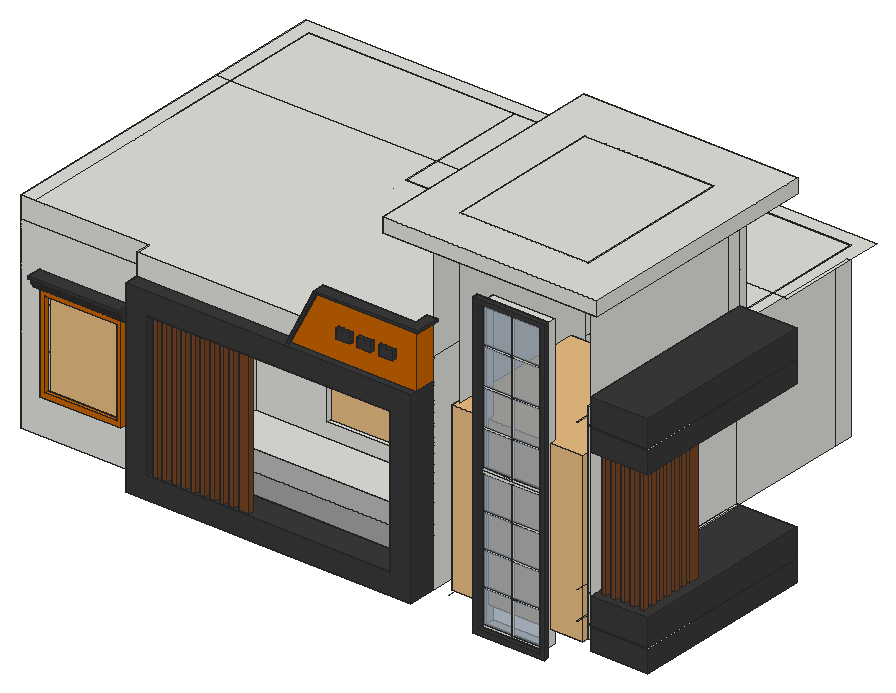
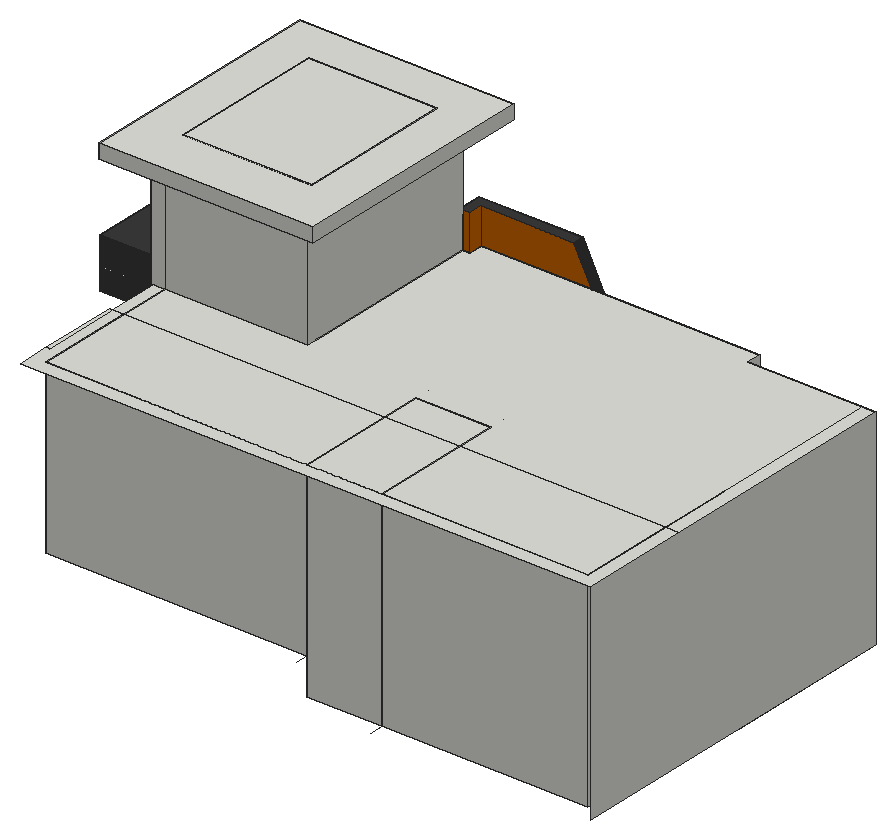
# SketchUp Ruby script. Lengths in inches.
U = 1.inch
M = Sketchup.active_model
def pt(a) = Geom::Point3d.new(a.map { |v| v * U })
def face(e, loops, mat)
  f = e.add_face(loops[0].map { |a| pt(a) })
  loops[1..].each { |l| e.add_face(l.map { |a| pt(a) }).erase! }
  f.material = f.back_material = mat if mat
  f
end
# faces: each face lists its corners as indices into pts; further lists are holes
def faces(e, pts, list, mat = nil) = list.each { |f| face(e, (f[0].is_a?(Array) ? f : [f]).map { |l| l.map { |i| pts[i] } }, mat) }
# xy, xz, yz: faces in a plane at the given z, y or x. An outline is a flat list of corners, or four numbers for a rectangle; further outlines are holes
def ring(l) = l.size == 4 ? [[l[0], l[1]], [l[2], l[1]], [l[2], l[3]], [l[0], l[3]]] : l.each_slice(2).to_a
def flat(e, list, mat, &to3) = list.each { |f| face(e, (f[0].is_a?(Array) ? f : [f]).map { |l| ring(l).map { |u, v| to3.(u, v) } }, mat) }
def xy(e, z, list, mat = nil) = flat(e, list, mat) { |x, y| [x, y, z] }
def xz(e, y, list, mat = nil) = flat(e, list, mat) { |x, z| [x, y, z] }
def yz(e, x, list, mat = nil) = flat(e, list, mat) { |y, z| [x, y, z] }
def lines(e, pts, list) = list.each { |a, b| e.add_line(pt(pts[a]), pt(pts[b])) }
# prism: a flat outline (further loops are holes) pulled along v
def prism(e, loops, v, mat = nil)
  f = face(e, loops, mat); d = Geom::Vector3d.new(v.map { |x| x * U })
  f.pushpull(f.normal.samedirection?(d) ? d.length : -d.length)
end
def box(e, o, s, mat = nil) = prism(e, [[o, [o[0] + s[0], o[1], o[2]], [o[0] + s[0], o[1] + s[1], o[2]], [o[0], o[1] + s[1], o[2]]]], [0, 0, s[2]], mat)
def at(x, y, z, deg = 0) = Geom::Transformation.translation(pt([x, y, z])) * Geom::Transformation.rotation(ORIGIN, Z_AXIS, deg.degrees)
def axes(o, x, y, z) = Geom::Transformation.new([*x, 0, *y, 0, *z, 0, *pt(o).to_a, 1])
def part(name) = M.definitions.add(name)
# library, detail: a bought-in or finely detailed component or shape, given as its bounding box
def library(name, o, s) = part(name).tap { |d| box(d.entities, o, s) }
def detail(e, o, s) = box(e.add_group.entities, o, s)
def put(e, d, t, mat = nil) = e.add_instance(d, t).tap { |i| i.material = mat if mat }
def group(e, t, mat = nil) = e.add_group.tap { |g| g.transformation = t; g.material = mat if mat }.entities
root = M.entities
M.materials.add("[Color C06]").color = [204, 102, 0]
M.materials.add("[Color M07]").color = [58, 58, 58]
M.materials.add("[Marble Carrara Floor Tile]").color = [204, 208, 219]
M.materials.add("[Modern Siding]").color = [191, 132, 100]
M.materials.add("[Polished Concrete New]").color = [200, 200, 203]
M.materials.add("[Stone Vein Gray]").color = [166, 165, 165]
M.materials.add("[Translucent Glass Sky Reflection]").color = [163, 177, 193]
M.materials["[Translucent Glass Sky Reflection]"].alpha = 0.52
M.materials.add("[Wood Floor]").color = [170, 81, 43]
M.materials.add("[Wood Veneer 01]").color = [120, 70, 37]
c1 = part("GLASS WINDOW")
g1 = group(c1.entities,at(60,0,0))
g2 = group(g1,at(-2,0.5,1.97),"[Translucent Glass Sky Reflection]")
box(g2,[-56,0,0],[56,0.75,114.1])
g3 = group(g1,at(0,0,0))
xy(g3,0,[[-60,0,0,2]])
xy(g3,1.97,[[-58,0,-58,2,-2,2,-2,0,-29.5,0,-29.5,1.25,-30.5,1.25,-30.5,0]])
xy(g3,29.75,[[-58,0,-30.5,1.25],[-29.5,0,-2,1.25]])
xy(g3,30.74,[[-58,0,-30.5,1.25],[-29.5,0,-2,1.25]])
xy(g3,58.52,[[-58,0,-30.5,1.25],[-29.5,0,-2,1.25]])
xy(g3,59.51,[[-58,0,-30.5,1.25],[-29.5,0,-2,1.25]])
xy(g3,87.29,[[-58,0,-30.5,1.25],[-29.5,0,-2,1.25]])
xy(g3,88.28,[[-58,0,-30.5,1.25],[-29.5,0,-2,1.25]])
xy(g3,116.0625,[[-58,0,-30.5,0,-30.5,1.25,-29.5,1.25,-29.5,0,-2,0,-2,2,-58,2]])
xy(g3,118.03,[[-60,0,0,2]])
xz(g3,0,[[[-60,0,0,118.03],[-58,59.51,-30.5,87.29],[-58,1.97,-30.5,29.75],[-58,88.28,-30.5,116.0625],[-58,30.74,-30.5,58.52],[-29.5,88.28,-2,116.0625],[-29.5,59.51,-2,87.29],[-29.5,1.97,-2,29.75],[-29.5,30.74,-2,58.52]]])
xz(g3,1.25,[[-30.5,1.97,-29.5,1.97,-29.5,29.75,-2,29.75,-2,30.74,-29.5,30.74,-29.5,58.52,-2,58.52,-2,59.51,-29.5,59.51,-29.5,87.29,-2,87.29,-2,88.28,-29.5,88.28,-29.5,116.0625,-30.5,116.0625,-30.5,88.28,-58,88.28,-58,87.29,-30.5,87.29,-30.5,59.51,-58,59.51,-58,58.52,-30.5,58.52,-30.5,30.74,-58,30.74,-58,29.75,-30.5,29.75]])
xz(g3,2,[[[-60,0,0,118.03],[-58,1.97,-2,116.0625]]])
yz(g3,-60,[[0,0,2,118.03]])
yz(g3,-58,[[0,1.97,0,29.75,1.25,29.75,1.25,30.74,0,30.74,0,58.52,1.25,58.52,1.25,59.51,0,59.51,0,87.29,1.25,87.29,1.25,88.28,0,88.28,0,116.0625,2,116.0625,2,1.97]])
yz(g3,-30.5,[[0,1.97,1.25,29.75],[0,30.74,1.25,58.52],[0,59.51,1.25,87.29],[0,88.28,1.25,116.0625]])
yz(g3,-29.5,[[0,1.97,1.25,29.75],[0,30.74,1.25,58.52],[0,59.51,1.25,87.29],[0,88.28,1.25,116.0625]])
yz(g3,-2,[[0,1.97,2,1.97,2,116.0625,0,116.0625,0,88.28,1.25,88.28,1.25,87.29,0,87.29,0,59.51,1.25,59.51,1.25,58.52,0,58.52,0,30.74,1.25,30.74,1.25,29.75,0,29.75]])
yz(g3,0,[[0,0,2,118.03]])
p = [[-29.5,0,116.0625],[-30.5,0,116.0625]]
lines(g3,p,[[0,1]])
c2 = library("DOG LEGGED STAIRCASE",[0,0,0],[168.93,78,123.9375])
c3 = library("Janela de Correr",[0,0,0],[62.99,2.6,47.24])
xy(root,121.92,[[359.58,113.36,409.62,113.6875]],"[Marble Carrara Floor Tile]")
xy(root,123.09,[[359.58,113.36,409.62,113.6875],[359.58,113.6875,409.62,121.61]],"[Marble Carrara Floor Tile]")
xy(root,126,[[384,20,444,24]],"[Color M07]")
xy(root,128.9,[[359.58,121.28,409.62,121.61]],"[Marble Carrara Floor Tile]")
xy(root,130,[[388,24,440,36]])
xy(root,130,[[388,20,440,24]],"[Color M07]")
xy(root,130.06,[[359.58,121.28,409.62,121.61],[359.58,121.61,409.62,129.53]],"[Marble Carrara Floor Tile]")
xy(root,132,[[24,120,48,184.5625]])
xy(root,135.87,[[359.58,129.2,409.62,129.53]],"[Marble Carrara Floor Tile]")
xy(root,137.03,[[359.58,129.2,409.62,129.53],[359.58,129.53,409.62,137.45]],"[Marble Carrara Floor Tile]")
xy(root,139.43,[[359.58,145.98,468,168]],"[Polished Concrete New]")
xy(root,142.84,[[359.58,137.12,409.62,137.45]],"[Marble Carrara Floor Tile]")
xy(root,144,[[0,24,12,168],[[12,24,12,120,204,120,204,36,192,36,192,24],[162,54,180,66]],[192,24,204,36],[204,24,348,156],[480,24,528,180],
  [468,36,477.125,180],[477.125,36,480,180],[12,120,204,153.875],[359.58,137.12,360,137.45],[359.58,137.45,360,168],
  [12,153.875,204,156],[12,156,348,168],[185.31,168,248.2,180],[348,168,468,180],[12,180,185.31,312],
  [185.31,180,248.2,184.3125],[185.31,184.3125,248.2,197.875],[185.31,197.875,248.2,312]])
xy(root,144,[[108,0,192,24],[192,0,204,24],[204,0,348,24]],"[Color M07]")
xy(root,144,[[360,137.12,409.62,137.45],[360,137.45,409.62,137.45,409.62,145.98,468,145.98,468,168,360,168]],"[Marble Carrara Floor Tile]")
xy(root,162,[[129,2,133,6],[145,2,149,6],[161,2,165,6],[185,2,189,6],[201,2,210,6],
  [126,24,330,48],[480,24,528,180],[126,48,330,114],[126,114,258,204],[258,114,330,114,330,144,328,144,328,148,330,148,330,188,328,188,328,192,330,192,330,204,324,204,324,199,320,199,320,204,273.87,204,273.87,199,270,199,270,204,258,204],
  [328,144,330,148],[328,188,330,192]])
xy(root,162,[[[126,0,330,24],[201,2,210,6],[193,2,197,6],[185,2,189,6],[177,2,181,6],[169,2,173,6],[161,2,165,6],[153,2,157,6],[145,2,149,6],[137,2,141,6],[129,2,133,6]]],"[Color M07]")
xy(root,163,[[480,24,528,180],[477.125,170.25,480,180]])
xy(root,174,[[186,114,246,204]])
xy(root,175.2,[[477.125,170.25,480,170.4375],[477.125,170.4375,480,180]])
xy(root,176,[[20,20,88,24]],"[Color C06]")
xy(root,180,[[24,24,84,143.1875]])
xy(root,180,[[24,20,84,24]],"[Color C06]")
xy(root,180,[[126,24,330,48]],"[Stone Vein Gray]")
xy(root,186,[[484,30,488,34],[500,30,504,34],[516,30,520,34],[516,46,520,50],[516,62,520,66],
  [516,78,520,86],[468,96,477.125,145.98],[477.125,96,480,170.4375],[468,145.98,477.125,168],[468,168,477.125,180],
  [477.125,170.4375,480,180]])
xy(root,186,[[[480,24,528,180],[516,78,520,86],[516,38,520,42],[492,30,496,34],[508,30,512,34],[516,46,520,50],[516,54,520,58],[516,62,520,66],[516,70,520,74],[484,30,488,34],[500,30,504,34],[516,30,520,34]]],"[Color M07]")
xy(root,237.2,[[328,148,330,188]])
xy(root,237.2,[[273.87,199,320,204]],"[Color M07]")
xy(root,241.2,[[186,114,246,204]])
xy(root,241.2,[[328,144,330,192],[270,199,324,204]],"[Color M07]")
xy(root,253.2,[[24,24,84,143.1875]])
xy(root,253.2,[[24,20,84,24]],"[Color C06]")
xy(root,257.2,[[20,20,88,24]],"[Color C06]")
xy(root,257.2,[[16,20,20,24],[88,20,92,24]],"[Color M07]")
xy(root,267.2,[[16,12,92,14]],"[Color M07]")
xy(root,269.2,[[16,12,92,24]],"[Color M07]")
xy(root,281.2,[[264,36,324,192]],"[Modern Siding]")
xy(root,283.2,[[[126,24,126,114,258,114,258,204,330,204,330,24],[264,36,324,192]],[264,36,324,192],[126,114,258,204]])
xy(root,283.2,[[126,0,330,24]],"[Color M07]")
xy(root,294,[[129,2,133,6],[137,2,141,6],[145,2,149,6],[153,2,157,6],[161,2,165,6],
  [169,2,173,6],[177,2,181,6],[185,2,189,6],[193,2,197,6],[201,2,210,6],
  [[480,24,528,180],[516,78,520,86],[516,38,520,42],[516,70,520,74],[516,62,520,66],[516,54,520,58],[516,46,520,50],[508,30,512,34],[492,30,496,34],[484,30,488,34],[516,30,520,34],[500,30,504,34]],[477.125,96,480,168],[477.125,168,480,180]])
xy(root,301.2,[[240,3,240,12,342,12,342,24,348,24,348,6,242.24,6,242.24,3],[108,12,342,24]])
xy(root,301.2,[[108,0,348,0,348,6,242.24,6,242.24,3,240,3,240,12,108,12]],"[Color M07]")
xy(root,312,[[480,24,528,180],[477.125,168,480,180]])
xy(root,313,[[480,24,528,180],[477.125,168,480,180]])
xy(root,319.2,[[108,12,342,12,342,24,348,24,348,187.0625,468,187.0625,468,230.125,248.2,230.125,248.2,197.875,185.31,197.875,185.31,230.125,12,230.125,12,24,108,24],[0,24,12,230.125],[468,36,477.125,187.0625],[477.125,168,480,180],[477.125,180,480,187.0625],
  [468,187.0625,477.125,230.125],[185.31,197.875,248.2,230.125],[0,230.125,12,230.125,12,312,468,312,468,230.125,477.125,230.125,477.125,296.25,480,296.25,480,324,0,324],[12,230.125,185.31,312],[185.31,230.125,248.2,312],
  [248.2,230.125,468,312],[477.125,230.125,480,296.25]])
xy(root,319.2,[[282,3,294,6],[300,3,312,6],[318,3,330,6]],"[Color M07]")
xy(root,327.2,[[282,3,294,6],[300,3,312,6],[318,3,330,6]],"[Color M07]")
xy(root,336,[[480,24,528,180]],"[Color M07]")
xy(root,347.2,[[265.24,3,351,6],[348,6,351,24]],"[Color M07]")
xy(root,349.2,[[264,3,351,3,351,24,342,24,342,12,264,12]],"[Color M07]")
xy(root,375.2,[[388,20,440,24],[388,24,440,36]])
xy(root,379.2,[[384,20,444,24]],"[Color M07]")
xy(root,414.2,[[[328,4,500,207.0625],[342,18,486,193.0625]]],"[Modern Siding]")
xy(root,415.2,[[[324,0,504,211.0625],[328,4,500,207.0625]],[[342,18,486,193.0625],[348,24,480,187.0625]],[[348,24,480,187.0625],[360,36,468,168]],[360,36,468,168]])
xy(root,427.2,[[[324,0,504,211.0625],[360,36,468,168]],[360,36,468,168]])
xz(root,0,[[324,415.2,504,427.2]])
xz(root,0,[[[108,144,348,301.2],[126,162,330,283.2]]],"[Color M07]")
xz(root,2,[[129,162,133,294],[137,162,141,294],[145,162,149,294],[153,162,157,294],[161,162,165,294],
  [169,162,173,294],[177,162,181,294],[185,162,189,294],[193,162,197,294],[201,162,210,294]],"[Wood Veneer 01]")
xz(root,3,[[240,301.2,242.24,301.2,265.24,347.2,351,347.2,351,349.2,264,349.2],[282,319.2,294,327.2],[300,319.2,312,327.2],[318,319.2,330,327.2]],"[Color M07]")
xz(root,4,[[328,414.2,500,415.2]],"[Modern Siding]")
xz(root,6,[[282,319.2,294,327.2],[318,319.2,330,327.2]])
xz(root,6,[[[242.24,301.2,348,301.2,348,347.2,265.24,347.2],[282,319.2,294,327.2],[300,319.2,312,327.2],[318,319.2,330,327.2]]],"[Color C06]")
xz(root,6,[[129,162,133,294],[137,162,141,294],[145,162,149,294],[153,162,157,294],[161,162,165,294],
  [169,162,173,294],[177,162,181,294],[185,162,189,294],[193,162,197,294],[201,162,210,294]],"[Wood Veneer 01]")
xz(root,12,[[108,301.2,240,301.2,249,319.2,108,319.2],[240,301.2,342,301.2,342,319.2,249,319.2]])
xz(root,12,[[249,319.2,264,349.2,342,349.2,342,319.2]],"[Color C06]")
xz(root,12,[[16,267.2,92,269.2]],"[Color M07]")
xz(root,18,[[342,414.2,486,415.2]],"[Modern Siding]")
xz(root,20,[[[20,176,88,257.2],[24,180,84,253.2]]],"[Color C06]")
xz(root,20,[[[384,126,444,379.2],[388,130,440,375.2]]],"[Color M07]")
xz(root,24,[[[384,126,444,379.2],[388,130,440,375.2]],[[0,144,108,301.2],[20,176,20,257.2,16,257.2,16,269.2,92,269.2,92,257.2,88,257.2,88,176]],[[108,144,348,301.2],[126,162,330,283.2]],[[20,176,88,257.2],[24,180,84,253.2]],[16,257.2,92,269.2],
  [0,301.2,108,319.2],[342,301.2,348,319.2],[348,347.2,351,349.2]])
xz(root,24,[[342,319.2,348,349.2]],"[Color C06]")
xz(root,24,[[480,144,528,162],[480,163,528,186],[480,294,528,312],[480,313,528,336]],"[Color M07]")
xz(root,24,[[126,162,330,180]],"[Stone Vein Gray]")
xz(root,30,[[484,186,488,294],[492,186,496,294],[500,186,504,294],[508,186,512,294],[516,186,520,294]],"[Wood Veneer 01]")
xz(root,34,[[484,186,488,294],[492,186,496,294],[500,186,504,294],[508,186,512,294],[516,186,520,294]],"[Wood Veneer 01]")
xz(root,36,[[468,144,477.125,319.2],[360,415.2,468,427.2]])
xz(root,36,[[264,281.2,324,283.2]],"[Modern Siding]")
xz(root,38,[[516,186,520,294]],"[Wood Veneer 01]")
xz(root,42,[[516,186,520,294]],"[Wood Veneer 01]")
xz(root,46,[[516,186,520,294]],"[Wood Veneer 01]")
xz(root,48,[[126,162,330,180]])
xz(root,50,[[516,186,520,294]],"[Wood Veneer 01]")
xz(root,54,[[516,186,520,294]],"[Wood Veneer 01]")
xz(root,58,[[516,186,520,294]],"[Wood Veneer 01]")
xz(root,62,[[516,186,520,294]],"[Wood Veneer 01]")
xz(root,66,[[516,186,520,294]],"[Wood Veneer 01]")
xz(root,70,[[516,186,520,294]],"[Wood Veneer 01]")
xz(root,74,[[516,186,520,294]],"[Wood Veneer 01]")
xz(root,78,[[516,186,520,294]],"[Wood Veneer 01]")
xz(root,86,[[516,186,520,294]],"[Wood Veneer 01]")
xz(root,96,[[477.125,186,480,294]])
xz(root,113.6875,[[359.58,121.92,409.62,123.09]],"[Marble Carrara Floor Tile]")
xz(root,114,[[[126,162,258,283.2],[186,174,246,241.2]]])
xz(root,120,[[60,143,108,144],[108,143,192.6875,144]],"[Color M07]")
xz(root,121.61,[[359.58,123.09,409.62,128.9],[359.58,128.9,409.62,130.06]],"[Marble Carrara Floor Tile]")
xz(root,129.53,[[359.58,130.06,409.62,135.87],[359.58,135.87,409.62,137.03]],"[Marble Carrara Floor Tile]")
xz(root,137.45,[[359.58,137.03,409.62,142.84],[359.58,142.84,409.62,144]],"[Marble Carrara Floor Tile]")
xz(root,143.1875,[[24,180,84,253.2]])
xz(root,144,[[328,162,330,241.2]],"[Color M07]")
xz(root,145.98,[[409.62,139.43,468,144]],"[Polished Concrete New]")
xz(root,148,[[328,162,330,237.2]])
xz(root,168,[[477.125,294,480,312],[477.125,312,480,313],[360,415.2,468,427.2]])
xz(root,170.25,[[477.125,163,480,175.2]])
xz(root,170.4375,[[477.125,175.2,480,186]])
xz(root,180,[[468,144,477.125,162],[477.125,144,480,163],[468,163,477.125,175.2],[477.125,163,480,175.2],[468,175.2,477.125,186],
  [477.125,175.2,480,186],[468,186,477.125,186.125],[468,186.125,477.125,294],[477.125,294,480,312],[477.125,313,480,319.2]])
xz(root,180,[[480,144,528,162],[480,163,528,175.2],[480,175.2,528,186],[480,294,528,312],[480,313,528,319.2],
  [480,319.2,528,336]],"[Color M07]")
xz(root,187.0625,[[348,319.2,468,415.2],[468,319.2,480,415.2]])
xz(root,188,[[328,162,330,237.2]],"[Color M07]")
xz(root,192,[[264,281.2,324,283.2]])
xz(root,192,[[328,162,330,241.2]],"[Color M07]")
xz(root,193.0625,[[342,414.2,486,415.2]],"[Modern Siding]")
xz(root,197.875,[[185.31,144,248.2,319.2]])
xz(root,199,[[270,162,273.87,162,273.87,237.2,320,237.2,320,162,324,162,324,241.2,270,241.2]],"[Color M07]")
xz(root,204,[[[126,162,258,283.2],[186,174,246,241.2]],[258,162,270,162,270,241.2,324,241.2,324,162,330,162,330,283.2,258,283.2]])
xz(root,204,[[273.87,162,320,237.2]],"[Wood Floor]")
xz(root,207.0625,[[328,414.2,500,415.2]],"[Modern Siding]")
xz(root,211.0625,[[324,415.2,504,427.2]])
xz(root,312,[[12,144,185.31,319.2],[185.31,144,248.2,319.2],[248.2,175.2,468,319.2]])
yz(root,0,[[24,144,324,319.2]])
yz(root,12,[[168,144,180,319.2],[180,144,312,319.2]])
yz(root,16,[[20,257.2,19.23,257.67,18.5,258.21,17.83,258.8125,17.21,259.48,16.67,260.2,16.1875,260.97,15.79,261.78,15.46,262.63,15.22,263.5,15.0625,264.39,14.99,265.29,15,266.2,14,267.2,12,267.2,12,269.2,24,269.2,24,257.2]],"[Color M07]")
yz(root,20,[[20,176,24,257.2]],"[Color C06]")
yz(root,24,[[24,180,143.1875,253.2]])
yz(root,24,[[20,180,24,253.2]],"[Color C06]")
yz(root,84,[[24,180,143.1875,253.2]])
yz(root,84,[[20,180,24,253.2]],"[Color C06]")
yz(root,88,[[20,176,24,257.2]],"[Color C06]")
yz(root,92,[[20,257.2,24,257.2,24,269.2,12,269.2,12,267.2,14,267.2,15,266.2,14.99,265.29,15.0625,264.39,15.22,263.5,15.46,262.63,15.79,261.78,16.1875,260.97,16.67,260.2,17.21,259.48,17.83,258.8125,18.5,258.21,19.23,257.67]],"[Color M07]")
yz(root,108,[[12,301.2,24,319.2]])
yz(root,108,[[0,144,24,301.2]],"[Color M07]")
yz(root,126,[[24,162,48,180],[48,162,114,162,114,283.2,24,283.2,24,180,48,180],[114,162,204,283.2]])
yz(root,126,[[0,162,24,283.2]],"[Color M07]")
yz(root,129,[[2,162,6,294]],"[Wood Veneer 01]")
yz(root,133,[[2,162,6,294]],"[Wood Veneer 01]")
yz(root,137,[[2,162,6,294]],"[Wood Veneer 01]")
yz(root,141,[[2,162,6,294]],"[Wood Veneer 01]")
yz(root,145,[[2,162,6,294]],"[Wood Veneer 01]")
yz(root,149,[[2,162,6,294]],"[Wood Veneer 01]")
yz(root,153,[[2,162,6,294]],"[Wood Veneer 01]")
yz(root,157,[[2,162,6,294]],"[Wood Veneer 01]")
yz(root,161,[[2,162,6,294]],"[Wood Veneer 01]")
yz(root,165,[[2,162,6,294]],"[Wood Veneer 01]")
yz(root,169,[[2,162,6,294]],"[Wood Veneer 01]")
yz(root,173,[[2,162,6,294]],"[Wood Veneer 01]")
yz(root,177,[[2,162,6,294]],"[Wood Veneer 01]")
yz(root,181,[[2,162,6,294]],"[Wood Veneer 01]")
yz(root,185,[[2,162,6,294]],"[Wood Veneer 01]")
yz(root,185.31,[[197.875,144,312,319.2]])
yz(root,186,[[114,174,204,241.2]])
yz(root,189,[[2,162,6,294]],"[Wood Veneer 01]")
yz(root,193,[[2,162,6,294]],"[Wood Veneer 01]")
yz(root,197,[[2,162,6,294]],"[Wood Veneer 01]")
yz(root,201,[[2,162,6,294]],"[Wood Veneer 01]")
yz(root,210,[[2,162,6,294]],"[Wood Veneer 01]")
yz(root,246,[[114,174,204,241.2]])
yz(root,248.2,[[184.3125,144,197.875,175.2],[197.875,144,312,175.2],[197.875,175.2,312,319.2]])
yz(root,258,[[114,162,204,283.2]])
yz(root,264,[[36,281.2,192,283.2]],"[Modern Siding]")
yz(root,270,[[199,162,204,241.2]],"[Color M07]")
yz(root,273.87,[[199,162,204,237.2]],"[Color M07]")
yz(root,282,[[3,319.2,6,327.2]],"[Color M07]")
yz(root,294,[[3,319.2,6,327.2]],"[Color M07]")
yz(root,300,[[3,319.2,6,327.2]],"[Color M07]")
yz(root,312,[[3,319.2,6,327.2]],"[Color M07]")
yz(root,318,[[3,319.2,6,327.2]],"[Color M07]")
yz(root,320,[[199,162,204,237.2]],"[Color M07]")
yz(root,324,[[0,415.2,211.0625,427.2]])
yz(root,324,[[199,162,204,241.2]],"[Color M07]")
yz(root,324,[[36,281.2,192,283.2]],"[Modern Siding]")
yz(root,328,[[144,162,144,241.2,192,241.2,192,162,188,162,188,237.2,148,237.2,148,162]],"[Color M07]")
yz(root,328,[[4,414.2,207.0625,415.2]],"[Modern Siding]")
yz(root,330,[[24,162,48,180],[48,162,48,180,24,180,24,283.2,204,283.2,204,162,192,162,192,241.2,144,241.2,144,162],[144,162,148,162,148,237.2,188,237.2,188,162,192,162,192,241.2,144,241.2]])
yz(root,330,[[0,162,24,283.2],[3,319.2,6,327.2]],"[Color M07]")
yz(root,330,[[148,162,188,237.2]],"[Wood Floor]")
yz(root,342,[[12,301.2,24,319.2]])
yz(root,342,[[12,319.2,24,349.2]],"[Color C06]")
yz(root,342,[[18,414.2,193.0625,415.2]],"[Modern Siding]")
yz(root,348,[[24,144,168,319.2],[168,144,180,319.2],[24,319.2,187.0625,415.2]])
yz(root,348,[[6,301.2,24,347.2]],"[Color C06]")
yz(root,348,[[0,144,24,301.2]],"[Color M07]")
yz(root,351,[[3,347.2,24,349.2]],"[Color M07]")
yz(root,359.58,[[113.36,121.92,113.27,121.94,113.19,122,113.12,122.09,113.07,122.21,113.04,122.35,113.03,122.51,113.04,122.66,113.07,122.8,113.12,122.92,113.19,123.01,113.27,123.07,113.36,123.09,113.6875,123.09,113.6875,121.92],[121.28,128.9,121.19,128.92,121.11,128.97,121.04,129.07,120.99,129.1875,120.96,129.33,120.95,129.48,120.96,129.625,120.99,129.77,121.04,129.89,121.11,129.98,121.19,130.04,121.28,130.06,121.61,130.06,121.61,128.9],[129.2,135.87,129.11,135.89,129.03,135.94,128.96,136.04,128.91,136.16,128.875,136.3,128.87,136.45,128.875,136.6,128.91,136.74,128.96,136.86,129.03,136.95,129.11,137.01,129.2,137.03,129.53,137.03,129.53,135.87],[137.12,142.84,137.03,142.86,136.95,142.92,136.88,143.01,136.83,143.13,136.8,143.27,136.79,143.42,136.8,143.57,136.83,143.71,136.88,143.83,136.95,143.92,137.03,143.98,137.12,144,137.45,144,137.45,142.84]],"[Marble Carrara Floor Tile]")
yz(root,360,[[36,144,168,415.2],[36,415.2,168,427.2]])
yz(root,384,[[20,126,24,379.2]],"[Color M07]")
yz(root,388,[[24,130,36,375.2]])
yz(root,388,[[20,130,24,375.2]],"[Color M07]")
yz(root,409.62,[[113.36,121.92,113.6875,121.92,113.6875,123.09,113.36,123.09,113.27,123.07,113.19,123.01,113.12,122.92,113.07,122.8,113.04,122.66,113.03,122.51,113.04,122.35,113.07,122.21,113.12,122.09,113.19,122,113.27,121.94],[121.28,128.9,121.61,128.9,121.61,130.06,121.28,130.06,121.19,130.04,121.11,129.98,121.04,129.89,120.99,129.77,120.96,129.625,120.95,129.48,120.96,129.33,120.99,129.1875,121.04,129.07,121.11,128.97,121.19,128.92],[129.2,135.87,129.53,135.87,129.53,137.03,129.2,137.03,129.11,137.01,129.03,136.95,128.96,136.86,128.91,136.74,128.875,136.6,128.87,136.45,128.875,136.3,128.91,136.16,128.96,136.04,129.03,135.94,129.11,135.89],[137.12,142.84,137.45,142.84,137.45,144,137.12,144,137.03,143.98,136.95,143.92,136.88,143.83,136.83,143.71,136.8,143.57,136.79,143.42,136.8,143.27,136.83,143.13,136.88,143.01,136.95,142.92,137.03,142.86]],"[Marble Carrara Floor Tile]")
yz(root,440,[[24,130,36,375.2]])
yz(root,440,[[20,130,24,375.2]],"[Color M07]")
yz(root,444,[[20,126,24,379.2]],"[Color M07]")
yz(root,468,[[145.98,139.43,168,144],[36,144,128.91,162],[128.91,144,129.53,162],[129.53,144,132,162],[132,144,137.45,162],
  [137.45,144,145.98,162],[145.98,144,168,162],[168,144,180,162],[36,162,128.91,163],[128.91,162,129.53,163],
  [129.53,162,132,163],[132,162,137.45,163],[137.45,162,145.98,163],[145.98,162,168,163],[168,162,180,163],
  [36,163,145.98,186.125],[128.91,163,129.53,186],[129.53,163,132,186],[132,163,137.45,186],[137.45,163,145.98,186.125],
  [145.98,163,168,186],[168,163,180,186],[180,175.2,296.25,319.2],[296.25,175.2,312,319.2],[128.91,186,129.53,186.125],
  [129.53,186,132,186.125],[132,186,137.45,186.125],[145.98,186,168,186.125],[168,186,180,186.125],[36,186.125,128.91,319.2],
  [128.91,186.125,129.53,319.2],[129.53,186.125,132,319.2],[132,186.125,137.45,319.2],[137.45,186.125,168,319.2],[168,186.125,180,319.2],
  [36,415.2,168,427.2]])
yz(root,477.125,[[36,144,180,163],[36,163,170.25,163,170.25,186,96,186,96,186.125,36,186.125],[170.25,163,180,175.2],[170.25,175.2,180,175.2,180,312,168,312,168,294,96,294,96,186,170.25,186],[170.25,175.2,170.4375,186],
  [170.4375,175.2,180,186],[96,186,170.25,186.125],[170.25,186,180,186.125],[36,186.125,96,186.125,96,294,168,294,168,313,36,313],[96,186.125,180,294],
  [168,294,180,312],[36,313,168.1875,319.2],[168.1875,313,180,319.2]])
yz(root,480,[[24,144,180,162],[24,162,180,163],[24,163,24,186,170.4375,186,170.4375,175.2,170.25,175.2,170.25,163],[170.25,163,180,175.2],[170.4375,175.2,180,186],
  [24,186,96,294],[24,294,168,312],[168,294,180,312],[24,312,168,313],[24,313,24,336,168,336,168,319.2,180,319.2,180,313],
  [168,319.2,180,336],[180,319.2,187.0625,415.2],[24,336,168,415.2],[168,336,180,415.2]])
yz(root,484,[[30,186,34,294]],"[Wood Veneer 01]")
yz(root,486,[[18,414.2,193.0625,415.2]],"[Modern Siding]")
yz(root,488,[[30,186,34,294]],"[Wood Veneer 01]")
yz(root,492,[[30,186,34,294]],"[Wood Veneer 01]")
yz(root,496,[[30,186,34,294]],"[Wood Veneer 01]")
yz(root,500,[[4,414.2,207.0625,415.2]],"[Modern Siding]")
yz(root,500,[[30,186,34,294]],"[Wood Veneer 01]")
yz(root,504,[[0,415.2,211.0625,427.2]])
yz(root,504,[[30,186,34,294]],"[Wood Veneer 01]")
yz(root,508,[[30,186,34,294]],"[Wood Veneer 01]")
yz(root,512,[[30,186,34,294]],"[Wood Veneer 01]")
yz(root,516,[[30,186,34,294],[38,186,42,294],[46,186,50,294],[54,186,58,294],[62,186,66,294],
  [70,186,74,294],[78,186,86,294]],"[Wood Veneer 01]")
yz(root,520,[[30,186,34,294],[38,186,42,294],[46,186,50,294],[54,186,58,294],[62,186,66,294],
  [70,186,74,294],[78,186,86,294]],"[Wood Veneer 01]")
yz(root,528,[[24,144,180,162],[24,163,180,186],[24,294,180,312],[24,313,180,336]],"[Color M07]")
p = [[359.58,113.19,122],[359.58,113.27,121.94],[409.62,113.27,121.94],[409.62,113.19,122],[359.58,113.36,121.92],[409.62,113.36,121.92],
  [359.58,113.12,122.09],[409.62,113.12,122.09],[359.58,113.07,122.21],[409.62,113.07,122.21],[359.58,113.04,122.35],[409.62,113.04,122.35],
  [359.58,113.03,122.51],[409.62,113.03,122.51],[359.58,113.04,122.66],[409.62,113.04,122.66],[359.58,113.07,122.8],[409.62,113.07,122.8],
  [359.58,113.12,122.92],[409.62,113.12,122.92],[359.58,113.19,123.01],[409.62,113.19,123.01],[359.58,113.27,123.07],[409.62,113.27,123.07],
  [359.58,113.36,123.09],[409.62,113.36,123.09],[359.58,121.11,128.97],[359.58,121.19,128.92],[409.62,121.19,128.92],[409.62,121.11,128.97],
  [359.58,121.28,128.9],[409.62,121.28,128.9],[359.58,121.04,129.07],[409.62,121.04,129.07],[359.58,120.99,129.1875],[409.62,120.99,129.1875],
  [359.58,120.96,129.33],[409.62,120.96,129.33],[359.58,120.95,129.48],[409.62,120.95,129.48],[359.58,120.96,129.625],[409.62,120.96,129.625],
  [359.58,120.99,129.77],[409.62,120.99,129.77],[359.58,121.04,129.89],[409.62,121.04,129.89],[359.58,121.11,129.98],[409.62,121.11,129.98],
  [359.58,121.19,130.04],[409.62,121.19,130.04],[359.58,121.28,130.06],[409.62,121.28,130.06],[359.58,129.03,135.94],[359.58,129.11,135.89],
  [409.62,129.11,135.89],[409.62,129.03,135.94],[359.58,128.96,136.04],[409.62,128.96,136.04],[359.58,129.2,135.87],[409.62,129.2,135.87],
  [359.58,128.91,136.16],[409.62,128.91,136.16],[359.58,128.875,136.3],[409.62,128.875,136.3],[359.58,128.87,136.45],[409.62,128.87,136.45],
  [359.58,128.875,136.6],[409.62,128.875,136.6],[359.58,128.91,136.74],[409.62,128.91,136.74],[359.58,128.96,136.86],[409.62,128.96,136.86],
  [359.58,129.03,136.95],[409.62,129.03,136.95],[359.58,129.11,137.01],[409.62,129.11,137.01],[359.58,129.2,137.03],[409.62,129.2,137.03],
  [359.58,137.03,142.86],[359.58,137.12,142.84],[409.62,137.12,142.84],[409.62,137.03,142.86],[359.58,136.88,143.01],[359.58,136.95,142.92],
  [409.62,136.95,142.92],[409.62,136.88,143.01],[359.58,136.83,143.13],[409.62,136.83,143.13],[359.58,136.8,143.27],[409.62,136.8,143.27],
  [359.58,136.79,143.42],[409.62,136.79,143.42],[359.58,136.8,143.57],[409.62,136.8,143.57],[359.58,136.83,143.71],[409.62,136.83,143.71],
  [359.58,136.88,143.83],[409.62,136.88,143.83],[359.58,136.95,143.92],[409.62,136.95,143.92],[359.58,137.03,143.98],[409.62,137.03,143.98],
  [359.58,137.12,144],[409.62,137.12,144],[360,137.12,144],[92,19.23,257.67],[16,19.23,257.67],[16,20,257.2],
  [20,20,257.2],[88,20,257.2],[92,20,257.2],[92,18.5,258.21],[16,18.5,258.21],[92,17.83,258.8125],
  [16,17.83,258.8125],[92,17.21,259.48],[16,17.21,259.48],[92,16.67,260.2],[16,16.67,260.2],[92,16.1875,260.97],
  [16,16.1875,260.97],[92,15.79,261.78],[16,15.79,261.78],[92,15.46,262.63],[16,15.46,262.63],[92,15.22,263.5],
  [16,15.22,263.5],[92,15.0625,264.39],[16,15.0625,264.39],[92,14.99,265.29],[16,14.99,265.29],[92,15,266.2],
  [16,15,266.2],[92,14,267.2],[16,14,267.2],[240,12,301.2],[240,3,301.2],[264,3,349.2],
  [264,12,349.2],[249,12,319.2],[242.24,6,301.2],[265.24,6,347.2],[265.24,3,347.2],[242.24,3,301.2],
  [360,36,144],[360,24,144],[248.2,324,175.2],[248.2,312,175.2],[185.31,312,144],[185.31,324,144],
  [477.125,96,294],[468,96,294],[468,24,313],[468,36,313],[477.125,180,313],[468,180,313],
  [468,36,312],[468,24,312],[468,36,163],[468,24,163],[248.2,184.3125,175.2],[248.2,184.3125,319.2],
  [185.31,184.3125,144],[185.31,184.3125,319.2],[468,36,162],[468,24,162],[468,36,186.125],[468,24,186.125],
  [477.125,36,162],[477.125,24,162],[477.125,36,312],[477.125,24,312],[477.125,36,186.125],[477.125,24,186.125],
  [477.125,36,163],[477.125,24,163],[477.125,36,313],[477.125,24,313]]
faces(root,p,[[0,1,2,3],[1,4,5,2],[6,0,3,7],[8,6,7,9],[10,8,9,11],[12,10,11,13],[14,12,13,15],[16,14,15,17],
  [18,16,17,19],[20,18,19,21],[22,20,21,23],[24,22,23,25],[26,27,28,29],[27,30,31,28],[32,26,29,33],[34,32,33,35],
  [36,34,35,37],[38,36,37,39],[40,38,39,41],[42,40,41,43],[44,42,43,45],[46,44,45,47],[48,46,47,49],[50,48,49,51],
  [52,53,54,55],[56,52,55,57],[53,58,59,54],[60,56,57,61],[62,60,61,63],[64,62,63,65],[66,64,65,67],[68,66,67,69],
  [70,68,69,71],[72,70,71,73],[74,72,73,75],[76,74,75,77],[78,79,80,81],[82,83,84,85],[83,78,81,84],[86,82,85,87],
  [88,86,87,89],[90,88,89,91],[92,90,91,93],[94,92,93,95],[96,94,95,97],[98,96,97,99],[100,98,99,101],[102,100,101,103,104]],"[Marble Carrara Floor Tile]")
faces(root,p,[[105,106,107,108,109,110],[111,112,106,105],[113,114,112,111],[115,116,114,113],[117,118,116,115],[119,120,118,117],[121,122,120,119],[123,124,122,121],
  [125,126,124,123],[127,128,126,125],[129,130,128,127],[131,132,130,129],[133,134,132,131],[135,136,137,138,139],[140,141,142,143]],"[Color M07]")
lines(root,p,[[144,145],[146,147],[148,149],[150,151],[152,153],[154,155],[156,157],[158,159],[160,161],[162,163],[164,165],[166,167],
  [168,169],[170,171],[172,173],[174,175],[176,177]])
put(root,c1,axes([388,24,130],[0.86778,0,0],[0,1,0],[0,0,1]))
put(root,c2,axes([467.46,30.6875,144],[0,0.72075,0],[-1.408,0,0],[0,0,1.12918]))
put(root,c3,axes([186,118.18,174],[0.94264,0,0],[0,0.63,0],[0,0,1.4224]))
put(root,c3,axes([24,24.6,180],[0.9525,0,0],[0,0.77,0],[0,0,1.5494]))
put(root,c1,axes([388,24,248.03],[0.86778,0,0],[0,1,0],[0,0,1.07741]))
